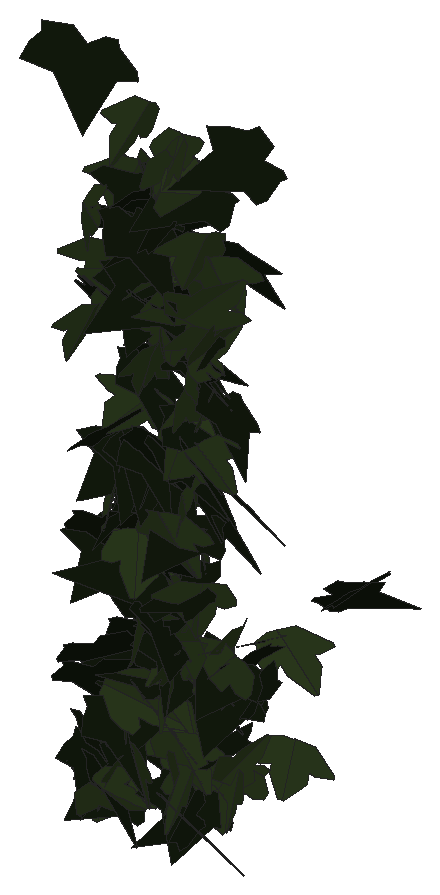
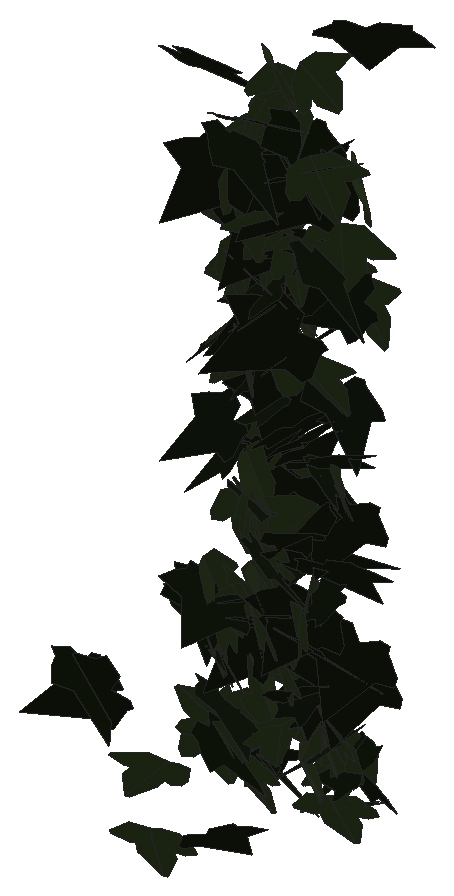
# SketchUp Ruby script. Lengths in inches.
U = 1.inch
M = Sketchup.active_model
def pt(a) = Geom::Point3d.new(a.map { |v| v * U })
def face(e, loops, mat)
  f = e.add_face(loops[0].map { |a| pt(a) })
  loops[1..].each { |l| e.add_face(l.map { |a| pt(a) }).erase! }
  f.material = f.back_material = mat if mat
  f
end
# faces: each face lists its corners as indices into pts; further lists are holes
def faces(e, pts, list, mat = nil) = list.each { |f| face(e, (f[0].is_a?(Array) ? f : [f]).map { |l| l.map { |i| pts[i] } }, mat) }
# xy, xz, yz: faces in a plane at the given z, y or x. An outline is a flat list of corners, or four numbers for a rectangle; further outlines are holes
def ring(l) = l.size == 4 ? [[l[0], l[1]], [l[2], l[1]], [l[2], l[3]], [l[0], l[3]]] : l.each_slice(2).to_a
def flat(e, list, mat, &to3) = list.each { |f| face(e, (f[0].is_a?(Array) ? f : [f]).map { |l| ring(l).map { |u, v| to3.(u, v) } }, mat) }
def xy(e, z, list, mat = nil) = flat(e, list, mat) { |x, y| [x, y, z] }
def xz(e, y, list, mat = nil) = flat(e, list, mat) { |x, z| [x, y, z] }
def yz(e, x, list, mat = nil) = flat(e, list, mat) { |y, z| [x, y, z] }
def lines(e, pts, list) = list.each { |a, b| e.add_line(pt(pts[a]), pt(pts[b])) }
# prism: a flat outline (further loops are holes) pulled along v
def prism(e, loops, v, mat = nil)
  f = face(e, loops, mat); d = Geom::Vector3d.new(v.map { |x| x * U })
  f.pushpull(f.normal.samedirection?(d) ? d.length : -d.length)
end
def box(e, o, s, mat = nil) = prism(e, [[o, [o[0] + s[0], o[1], o[2]], [o[0] + s[0], o[1] + s[1], o[2]], [o[0], o[1] + s[1], o[2]]]], [0, 0, s[2]], mat)
def at(x, y, z, deg = 0) = Geom::Transformation.translation(pt([x, y, z])) * Geom::Transformation.rotation(ORIGIN, Z_AXIS, deg.degrees)
def axes(o, x, y, z) = Geom::Transformation.new([*x, 0, *y, 0, *z, 0, *pt(o).to_a, 1])
def part(name) = M.definitions.add(name)
# library, detail: a bought-in or finely detailed component or shape, given as its bounding box
def library(name, o, s) = part(name).tap { |d| box(d.entities, o, s) }
def detail(e, o, s) = box(e.add_group.entities, o, s)
def put(e, d, t, mat = nil) = e.add_instance(d, t).tap { |i| i.material = mat if mat }
def group(e, t, mat = nil) = e.add_group.tap { |g| g.transformation = t; g.material = mat if mat }.entities
root = M.entities
M.materials.add("1026 AP 7946 SUNNY SIDE UP").color = [254, 231, 186]
M.materials.add("efeu1").color = [18, 25, 13]
M.materials.add("efeu2").color = [43, 57, 29]
c1 = part("ivyleaf_10")
p = [[0,0.5,-0.03],[-0.0625,2.02,-0.43],[-0.19,2.01,-0.46],[-0.54,1.05,-0.29],[-0.52,0.625,-0.18],[-0.83,0.76,-0.28],
  [-1.16,0.64,-0.33],[-1.15,0.33,-0.24],[-0.77,-0.39,0.02],[-0.3,-0.51,0.16],[0.04,-0.48,0.23],[-0.02,2.01,-0.4375],
  [-0.06,2.01,-0.43],[0.04,-0.49,0.23],[0.67,-0.49,0.14],[1.38,0.36,-0.2],[1.375,0.51,-0.24],[0.81,0.65,-0.19],
  [0.62,0.59,-0.15],[0.6,1.09,-0.28],[0.5,1.23,-0.31]]
faces(c1.entities,p,[[0,1,2,3,4,5,6,7,8,9,10],[11,12,0,13,14,15,16,17,18,19,20]],"efeu2")
c2 = part("ivyleaf_9")
p = [[1.54,2.16,1.25],[1.36,2.04,1.19],[-0.21,0.99,0.68],[-0.71,1.11,0.82],[-0.85,0.86,0.67],[-0.8,0.17,0.21],
  [-0.9,-0.01,0.1],[-0.67,-0.16,-0.02],[-0.08,-0.08,-0.05],[-0.03,-0.6,-0.4],[0.65,-0.88,-0.66],[0.83,-0.6,-0.49],
  [1.29,-0.42,-0.43],[1.8125,-0.07,-0.26],[1.21,0.44,0.15]]
faces(c2.entities,p,[[0,1,2,3,4,5,6,7,8,9,10,11,12,13,14]],"efeu1")
put(root,c1,axes([132.02,212.25,286.58],[-0.05135,-0.32161,0.09577],[-0.00011,-0.09523,-0.33345],[0.52721,-0.03135,0.00926]),"1026 AP 7946 SUNNY SIDE UP")
put(root,c2,axes([131.72,212.72,280.17],[0.23766,-0.27259,0.07051],[0.04751,-0.06328,-0.32145],[0.43998,0.15408,-0.00338]),"1026 AP 7946 SUNNY SIDE UP")
put(root,c2,axes([131.95,212.53,280.05],[-0.36569,-0.03792,-0.21571],[0.33427,-0.04152,-0.23598],[-0.00004,-0.31003,0.05612]),"1026 AP 7946 SUNNY SIDE UP")
put(root,c2,axes([131.95,212.3,290.48],[-0.32441,-0.28353,-0.12306],[0.1362,0.08246,-0.36015],[0.46319,-0.22283,0.01971]),"1026 AP 7946 SUNNY SIDE UP")
put(root,c2,axes([132.16,212.8125,282.98],[-0.45442,-0.14963,-0.00161],[0.02273,-0.02637,-0.33398],[0.23418,-0.28779,0.02929]),"1026 AP 7946 SUNNY SIDE UP")
put(root,c1,axes([132.15,212.54,280.18],[-0.41934,0.16198,0.05456],[-0.10293,-0.00838,-0.31876],[-0.24692,-0.27159,0.04022]),"1026 AP 7946 SUNNY SIDE UP")
put(root,c2,axes([132.0625,212.35,281.6875],[0.31074,0.29545,0.0152],[0.03651,0.00018,-0.36565],[-0.46358,0.19805,-0.01861]),"1026 AP 7946 SUNNY SIDE UP")
put(root,c2,axes([132.08,212.34,281.35],[0.36124,0.26486,-0.06174],[-0.0379,-0.06028,-0.36091],[-0.42584,0.23004,-0.02026]),"1026 AP 7946 SUNNY SIDE UP")
put(root,c2,axes([132.36,212.8125,287.3125],[-0.22975,0.30735,-0.01552],[-0.01057,-0.02179,-0.35036],[-0.48389,-0.14546,0.01502]),"1026 AP 7946 SUNNY SIDE UP")
put(root,c1,axes([132.12,212.73,279.58],[0.44585,0.09317,-0.07707],[-0.09975,-0.04747,-0.30671],[-0.15984,0.28952,-0.02357]),"1026 AP 7946 SUNNY SIDE UP")
put(root,c2,axes([132.21,212.71,279.47],[-0.35832,-0.15308,0.14069],[-0.03993,-0.1826,-0.25397],[0.321,-0.19359,0.12545]),"1026 AP 7946 SUNNY SIDE UP")
put(root,c1,axes([132.22,212.48,287.49],[-0.44394,-0.20665,0.02238],[0.00129,-0.03973,-0.35912],[0.32693,-0.28046,0.03181]),"1026 AP 7946 SUNNY SIDE UP")
put(root,c1,axes([131.95,212.37,288.07],[-0.01995,-0.10709,-0.34621],[0.18955,-0.31671,0.09761],[-0.52023,-0.11128,0.04884]),"1026 AP 7946 SUNNY SIDE UP")
put(root,c2,axes([131.85,212.55,286.74],[0.47745,-0.13961,0.0747],[0.09659,-0.04177,-0.34431],[0.22835,0.30956,-0.01056]),"1026 AP 7946 SUNNY SIDE UP")
put(root,c2,axes([131.97,212.81,280.53],[0.25597,-0.24314,-0.1334],[-0.01892,0.14245,-0.29343],[0.43172,0.1504,0.06623]),"1026 AP 7946 SUNNY SIDE UP")
put(root,c2,axes([132.26,215.04,280.1],[-0.30286,-0.23342,0.06508],[-0.05105,-0.05678,-0.3119],[0.37735,-0.19502,0.01004]),"1026 AP 7946 SUNNY SIDE UP")
put(root,c1,axes([132.32,212.83,288.57],[-0.30014,-0.2696,0.11055],[-0.02946,-0.11852,-0.33699],[0.4562,-0.18502,0.05097]),"1026 AP 7946 SUNNY SIDE UP")
put(root,c1,axes([132.21,212.7,280.64],[0.36739,-0.19883,0.07693],[0.06638,-0.06703,-0.31556],[0.32794,0.23632,-0.02231]),"1026 AP 7946 SUNNY SIDE UP")
put(root,c1,axes([132.19,212.5625,284.08],[0.26307,-0.2541,0.13388],[0.12807,-0.1036,-0.31385],[0.43119,0.1858,0.01154]),"1026 AP 7946 SUNNY SIDE UP")
put(root,c2,axes([132.39,212.81,284.39],[-0.37529,-0.19569,0.12924],[-0.06844,-0.14054,-0.30925],[0.36,-0.23072,0.07593]),"1026 AP 7946 SUNNY SIDE UP")
put(root,c2,axes([132.23,212.34,283.59],[0.40729,0.2018,-0.06657],[-0.05299,-0.06335,-0.33734],[-0.3295,0.25963,-0.02804]),"1026 AP 7946 SUNNY SIDE UP")
put(root,c2,axes([132.45,212.13,285.125],[0.01756,0.35128,0.00473],[-0.00169,0.00264,-0.36206],[-0.55237,0.01116,0.00126]),"1026 AP 7946 SUNNY SIDE UP")
put(root,c1,axes([132.54,212.4,287.0625],[-0.46318,-0.07603,0.15402],[-0.20051,-0.09607,-0.30884],[0.17226,-0.31626,0.05466]),"1026 AP 7946 SUNNY SIDE UP")
put(root,c1,axes([132.35,212.98,280.15],[0.22755,-0.24323,0.13062],[0.08195,-0.11795,-0.2919],[0.42447,0.15316,-0.01367]),"1026 AP 7946 SUNNY SIDE UP")
put(root,c1,axes([132.38,212.7,280.51],[-0.06852,0.28961,-0.11758],[-0.02646,-0.11891,-0.30061],[-0.4897,-0.0341,0.03269]),"1026 AP 7946 SUNNY SIDE UP")
put(root,c2,axes([132.17,212.6,282.51],[0.36831,-0.22817,-0.05604],[-0.03262,0.05459,-0.33562],[0.36691,0.23389,0.02641]),"1026 AP 7946 SUNNY SIDE UP")
put(root,c1,axes([132.48,212.3,280.1],[0.14974,-0.29281,0.1003],[0.03245,-0.09736,-0.3176],[0.48494,0.09693,-0.00972]),"1026 AP 7946 SUNNY SIDE UP")
put(root,c2,axes([132.24,212.32,279.87],[0.17493,-0.28596,0.10045],[0.03627,-0.0973,-0.31638],[0.47451,0.11286,-0.01285]),"1026 AP 7946 SUNNY SIDE UP")
put(root,c2,axes([132.36,212.47,280.75],[-0.00677,-0.32176,-0.09337],[-0.00453,0.08884,-0.33096],[0.52483,-0.00338,-0.00406]),"1026 AP 7946 SUNNY SIDE UP")
put(root,c1,axes([132.76,212.55,285.47],[-0.39866,-0.08442,0.21242],[-0.22566,-0.17792,-0.25729],[0.26889,-0.27448,0.09901]),"1026 AP 7946 SUNNY SIDE UP")
put(root,c2,axes([132.93,212.65,281.57],[-0.44466,0.1018,0.12948],[-0.21294,-0.01268,-0.30479],[-0.13778,-0.30897,0.05316]),"1026 AP 7946 SUNNY SIDE UP")
put(root,c1,axes([132.44,211.96,279.91],[-0.20154,-0.17471,-0.26525],[0.26771,0.19242,-0.22155],[0.40798,-0.21257,0.01435]),"1026 AP 7946 SUNNY SIDE UP")
put(root,c1,axes([132.65,212.82,282.05],[-0.36112,0.22578,0.02973],[-0.08714,-0.01754,-0.32767],[-0.34687,-0.23065,0.05137]),"1026 AP 7946 SUNNY SIDE UP")
put(root,c2,axes([132.68,212.48,284.1875],[-0.37109,0.09266,-0.2236],[0.26451,-0.15026,-0.25478],[-0.26135,-0.28365,0.05962]),"1026 AP 7946 SUNNY SIDE UP")
put(root,c2,axes([132.57,212.71,284.49],[-0.16532,-0.3031,0.0933],[-0.0495,-0.08676,-0.33101],[0.49574,-0.10974,-0.00194]),"1026 AP 7946 SUNNY SIDE UP")
put(root,c2,axes([133.03,212.61,282.82],[-0.3856,-0.01037,0.27824],[-0.4146,-0.07134,-0.24982],[0.09384,-0.35781,0.03957]),"1026 AP 7946 SUNNY SIDE UP")
put(root,c2,axes([132.61,212.81,288.4],[-0.29764,-0.27188,0.10545],[0.01456,-0.1295,-0.33248],[0.45742,-0.17279,0.0792]),"1026 AP 7946 SUNNY SIDE UP")
put(root,c1,axes([132.67,212.5,289.67],[-0.0965,-0.28665,0.21499],[0.04521,-0.21673,-0.29693],[0.5572,-0.03206,0.06133]),"1026 AP 7946 SUNNY SIDE UP")
put(root,c2,axes([132.63,212.87,281.05],[-0.2855,-0.26169,0.00417],[0.05023,-0.02884,-0.32534],[0.4085,-0.17935,0.04292]),"1026 AP 7946 SUNNY SIDE UP")
put(root,c2,axes([132.54,212.37,288.24],[0.44916,0.20282,0.03128],[0.06749,-0.01022,-0.35936],[-0.31506,0.28696,-0.03239]),"1026 AP 7946 SUNNY SIDE UP")
put(root,c2,axes([132.59,212.61,282.09],[0.39357,0.21173,0.01409],[0.04462,-0.01431,-0.33648],[-0.33051,0.2502,-0.02865]),"1026 AP 7946 SUNNY SIDE UP")
put(root,c2,axes([132.92,212.3125,288.7],[0.02627,0.34811,-0.02125],[0.00129,-0.02267,-0.35916],[-0.54852,0.01662,-0.00186]),"1026 AP 7946 SUNNY SIDE UP")
put(root,c2,axes([132.68,212.7,284.57],[-0.11155,-0.31917,0.08866],[-0.00763,-0.08886,-0.33704],[0.52048,-0.06971,0.01406]),"1026 AP 7946 SUNNY SIDE UP")
put(root,c1,axes([132.72,212.41,283.38],[0.34118,0.25212,-0.04792],[-0.0265,-0.04866,-0.34242],[-0.40267,0.21682,-0.01807]),"1026 AP 7946 SUNNY SIDE UP")
put(root,c2,axes([132.55,212.67,281.03],[0.40568,-0.18479,-0.0143],[-0.03477,-0.00888,-0.32633],[0.28918,0.25817,-0.01918]),"1026 AP 7946 SUNNY SIDE UP")
put(root,c1,axes([132.8,212.47,288.87],[-0.26253,0.3004,0.00141],[-0.01415,-0.00539,-0.35392],[-0.47213,-0.16688,0.00982]),"1026 AP 7946 SUNNY SIDE UP")
put(root,c1,axes([132.41,212.43,281.05],[0.08597,0.06552,0.35402],[0.51308,0.11482,-0.07544],[-0.19672,0.32809,-0.04206]),"1026 AP 7946 SUNNY SIDE UP")
put(root,c1,axes([132.88,212.57,287.12],[-0.14141,-0.3283,-0.00579],[0.02702,-0.00082,-0.35025],[0.51554,-0.09001,0.01677]),"1026 AP 7946 SUNNY SIDE UP")
put(root,c1,axes([132.65,212.53,282.02],[0.0263,0.01348,0.37394],[0.3193,-0.30153,0.00013],[0.4734,0.20263,-0.02086]),"1026 AP 7946 SUNNY SIDE UP")
put(root,c2,axes([132.84,212.61,287.16],[-0.28808,-0.28899,0.02913],[0.00038,-0.03552,-0.35216],[0.45684,-0.18221,0.01866]),"1026 AP 7946 SUNNY SIDE UP")
put(root,c1,axes([132.63,212.6,283.5],[0.33728,0.20601,0.16568],[0.18093,0.11068,-0.30574],[-0.36772,0.24342,0.00154]),"1026 AP 7946 SUNNY SIDE UP")
put(root,c2,axes([133.09,212.47,287.2],[-0.48227,-0.13072,0.09985],[-0.11533,-0.07531,-0.34157],[0.2292,-0.31295,0.03823]),"1026 AP 7946 SUNNY SIDE UP")
put(root,c2,axes([132.6875,212.68,285.83],[0.04918,-0.34284,0.00206],[-0.00195,-0.00407,-0.35467],[0.53911,0.03126,-0.00147]),"1026 AP 7946 SUNNY SIDE UP")
put(root,c2,axes([132.66,212.6,288.14],[0.50373,0.14468,0.03593],[0.07065,-0.01713,-0.36053],[-0.22277,0.32171,-0.03309]),"1026 AP 7946 SUNNY SIDE UP")
put(root,c1,axes([132.83,212.24,280.37],[-0.27438,0.24669,-0.08135],[0.04041,-0.07994,-0.31075],[-0.40596,-0.1747,0.02405]),"1026 AP 7946 SUNNY SIDE UP")
put(root,c2,axes([132.55,212.67,283.3],[0.12724,-0.13399,0.34566],[0.25159,-0.29587,-0.16284],[0.5106,0.17917,-0.0059]),"1026 AP 7946 SUNNY SIDE UP")
put(root,c2,axes([132.77,212.72,284.71],[-0.01177,-0.3344,-0.05727],[-0.00083,0.05372,-0.34426],[0.53254,-0.00731,-0.0018]),"1026 AP 7946 SUNNY SIDE UP")
put(root,c1,axes([132.88,212.86,281.38],[0.33985,-0.23052,0.05338],[0.06294,-0.03528,-0.32571],[0.36661,0.21975,0.00644]),"1026 AP 7946 SUNNY SIDE UP")
put(root,c1,axes([132.87,212.89,280.42],[0.18134,0.28609,-0.04332],[-0.01355,-0.0436,-0.31792],[-0.45486,0.11536,-0.0078]),"1026 AP 7946 SUNNY SIDE UP")
put(root,c2,axes([132.7,212.82,286.125],[0.49959,0.14204,0.13463],[0.20268,0.02912,-0.35749],[-0.22474,0.34201,-0.02312]),"1026 AP 7946 SUNNY SIDE UP")
put(root,c2,axes([132.66,212.57,283.43],[-0.0276,0.01244,0.34803],[0.36805,-0.24354,0.02034],[0.38338,0.23469,0.00552]),"1026 AP 7946 SUNNY SIDE UP")
put(root,c1,axes([133.07,212.23,286.4],[-0.00791,-0.34904,-0.0091],[0.00657,0.00679,-0.35955],[0.5489,-0.00511,0.00417]),"1026 AP 7946 SUNNY SIDE UP")
put(root,c2,axes([132.83,212.19,288.26],[0.11329,-0.34626,-0.11686],[-0.00785,0.11268,-0.36326],[0.57192,0.07014,0.01816]),"1026 AP 7946 SUNNY SIDE UP")
put(root,c2,axes([132.67,212.43,286.79],[0.48405,-0.08066,0.14025],[0.18948,-0.07502,-0.32586],[0.16221,0.32832,-0.03787]),"1026 AP 7946 SUNNY SIDE UP")
put(root,c2,axes([133.28,212.27,288.38],[-0.39014,0.19727,-0.1389],[0.11506,-0.12396,-0.32362],[-0.35871,-0.25431,0.04726]),"1026 AP 7946 SUNNY SIDE UP")
put(root,c1,axes([133.04,212.96,280.76],[0.06671,-0.3104,-0.01636],[0.00849,-0.01351,0.32265],[-0.48851,-0.04262,0.00337]),"1026 AP 7946 SUNNY SIDE UP")
put(root,c1,axes([133,212.86,287.63],[0.28652,0.28795,0.03353],[0.04248,0.01946,-0.3507],[-0.45339,0.1838,-0.01167]),"1026 AP 7946 SUNNY SIDE UP")
put(root,c2,axes([133.15,212.37,285.04],[0.45515,0.12855,-0.14607],[-0.1758,-0.09668,-0.32434],[-0.2453,0.30782,-0.03858]),"1026 AP 7946 SUNNY SIDE UP")
put(root,c2,axes([133.45,212.61,282.7],[-0.36608,0.23419,-0.01894],[-0.00426,-0.03042,-0.33952],[-0.36952,-0.23166,0.02268]),"1026 AP 7946 SUNNY SIDE UP")
put(root,c1,axes([133,215.08,280.83],[0.31959,0.20062,0.14624],[0.1968,0.07233,-0.29185],[-0.33136,0.23644,-0.03229]),"1026 AP 7946 SUNNY SIDE UP")
put(root,c1,axes([133.23,212.19,286.54],[0.09641,-0.29838,-0.17621],[0.06062,0.17694,-0.30574],[0.53606,0.03365,0.06626]),"1026 AP 7946 SUNNY SIDE UP")
put(root,c1,axes([133.23,212.85,281.76],[0.32329,-0.24763,-0.01854],[0.0259,0.03511,-0.3294],[0.38938,0.20326,0.0373]),"1026 AP 7946 SUNNY SIDE UP")
put(root,c1,axes([133.3125,212.86,284.08],[-0.00162,-0.32701,0.04336],[-0.00702,-0.04393,-0.33711],[0.51876,-0.00162,-0.00443]),"1026 AP 7946 SUNNY SIDE UP")
put(root,c1,axes([133.5,212.43,282.22],[0.28332,-0.06038,-0.27638],[-0.32867,0.17774,-0.18503],[0.28016,0.26956,0.06244]),"1026 AP 7946 SUNNY SIDE UP")
put(root,c2,axes([133.02,212.77,286.4],[0.22117,-0.29926,-0.09639],[0.00006,0.10073,-0.33739],[0.49223,0.13445,0.04335]),"1026 AP 7946 SUNNY SIDE UP")
put(root,c1,axes([133.27,212.56,287.23],[-0.15771,-0.33258,-0.04397],[0.09241,0.02446,-0.35416],[0.5187,-0.10548,0.04972]),"1026 AP 7946 SUNNY SIDE UP")
put(root,c2,axes([133.27,212.83,281.83],[-0.32737,-0.24699,-0.00352],[0.06004,-0.02958,-0.32922],[0.38371,-0.20609,0.04851]),"1026 AP 7946 SUNNY SIDE UP")
put(root,c1,axes([133.36,212.36,281.97],[0.02794,-0.32837,-0.10644],[-0.02402,0.10074,-0.33805],[0.53988,0.02147,-0.00953]),"1026 AP 7946 SUNNY SIDE UP")
put(root,c2,axes([133.125,212.52,282.26],[-0.06001,-0.26996,0.20533],[0.06915,-0.2044,-0.27562],[0.52454,-0.00394,0.05982]),"1026 AP 7946 SUNNY SIDE UP")
put(root,c2,axes([133,212.74,286.67],[0.30951,-0.28317,0.01911],[0.04012,-0.00678,-0.35488],[0.44458,0.19775,0.01872]),"1026 AP 7946 SUNNY SIDE UP")
put(root,c1,axes([133.17,212.44,281.53],[0.28084,-0.1946,0.18575],[0.19,-0.13532,-0.27289],[0.37268,0.21563,-0.00085]),"1026 AP 7946 SUNNY SIDE UP")
put(root,c1,axes([133.4,212.33,286.92],[-0.42699,-0.20649,0.02993],[-0.01226,-0.03954,-0.3506],[0.32791,-0.27035,0.02587]),"1026 AP 7946 SUNNY SIDE UP")
put(root,c2,axes([133.0625,212.68,286.16],[0.52825,-0.08164,0.00723],[0.00112,-0.02865,-0.35519],[0.1289,0.33481,-0.02654]),"1026 AP 7946 SUNNY SIDE UP")
put(root,c2,axes([133.59,212.9,288.625],[-0.17487,0.32529,-0.03444],[-0.01255,-0.03994,-0.35377],[-0.51434,-0.10962,0.02034]),"1026 AP 7946 SUNNY SIDE UP")
put(root,c1,axes([133.26,212.64,280.52],[-0.44557,-0.06004,-0.11776],[0.19649,-0.06127,-0.28719],[0.04917,-0.29922,0.08054]),"1026 AP 7946 SUNNY SIDE UP")
put(root,c1,axes([133.29,212.37,289.3125],[-0.1644,-0.29117,-0.2125],[0.19161,0.17108,-0.31395],[0.52576,-0.1534,0.04796]),"1026 AP 7946 SUNNY SIDE UP")
put(root,c2,axes([133.1,212.5,284.92],[0.32812,-0.25188,-0.09606],[-0.02957,0.10231,-0.33258],[0.42051,0.20373,0.05157]),"1026 AP 7946 SUNNY SIDE UP")
put(root,c1,axes([133.36,212.36,289.45],[0.37341,-0.26371,0.03526],[0.00857,-0.04304,-0.36496],[0.41836,0.23626,-0.02399]),"1026 AP 7946 SUNNY SIDE UP")
put(root,c2,axes([133.28,212.47,287.23],[0.32044,0.25277,0.11024],[0.11616,0.076,-0.33391],[-0.41477,0.21657,-0.00834]),"1026 AP 7946 SUNNY SIDE UP")
put(root,c1,axes([133.4,212.7,282.21],[0.23272,-0.29533,0.01306],[-0.00202,-0.0167,-0.3403],[0.46493,0.14776,-0.00801]),"1026 AP 7946 SUNNY SIDE UP")
put(root,c2,axes([133.69,212.67,286.72],[-0.4756,0.17076,-0.00236],[-0.01941,-0.02846,-0.35658],[-0.26785,-0.30114,0.03002]),"1026 AP 7946 SUNNY SIDE UP")
put(root,c1,axes([133.47,212.19,280.3],[0.16899,-0.25811,-0.19591],[-0.06551,0.18608,-0.28556],[0.49847,0.11196,0.02889]),"1026 AP 7946 SUNNY SIDE UP")
put(root,c2,axes([133.64,212.39,279.7],[-0.40245,0.17614,-0.03907],[0.03322,-0.03783,-0.3197],[-0.28169,-0.25611,0.01812]),"1026 AP 7946 SUNNY SIDE UP")
put(root,c1,axes([133.5,212.83,279.74],[0.42305,-0.12728,-0.10434],[-0.1553,0.02595,-0.30592],[0.20233,0.28605,-0.01666]),"1026 AP 7946 SUNNY SIDE UP")
put(root,c2,axes([133.61,212.7,288.79],[-0.51234,-0.1106,0.06176],[-0.01869,-0.14016,-0.33029],[0.1974,-0.30032,0.12903]),"1026 AP 7946 SUNNY SIDE UP")
put(root,c1,axes([133.48,212.4375,282.82],[0.37271,-0.20599,-0.11165],[-0.06278,0.11476,-0.31743],[0.3597,0.23347,0.06028]),"1026 AP 7946 SUNNY SIDE UP")
put(root,c2,axes([133.44,212.67,279.81],[-0.29395,-0.25273,-0.01862],[0.03919,0.00222,-0.32326],[0.39631,-0.18767,0.01816]),"1026 AP 7946 SUNNY SIDE UP")
put(root,c1,axes([133.4,214.71,279.54],[0.47351,0.07925,-0.01677],[-0.01939,-0.01879,-0.32053],[-0.12587,0.30102,-0.0137]),"1026 AP 7946 SUNNY SIDE UP")
put(root,c1,axes([133.3,212.55,281.5],[0.47852,0.05678,0.0851],[0.11727,0.04665,-0.31704],[-0.10469,0.31178,0.03387]),"1026 AP 7946 SUNNY SIDE UP")
put(root,c2,axes([133.29,212.84,281.5],[0.47461,-0.0762,-0.07099],[-0.11359,-0.00725,-0.31978],[0.11422,0.30942,-0.02306]),"1026 AP 7946 SUNNY SIDE UP")
put(root,c1,axes([133.41,212.16,284.02],[-0.4909,0.02305,-0.12555],[0.18611,-0.04446,-0.32094],[-0.05896,-0.33223,0.03225]),"1026 AP 7946 SUNNY SIDE UP")
put(root,c2,axes([133.62,212.42,284.08],[-0.5107,-0.11036,-0.06163],[0.10747,-0.01832,-0.35123],[0.16502,-0.32963,0.038]),"1026 AP 7946 SUNNY SIDE UP")
put(root,c1,axes([133.57,212.6875,283.51],[-0.19314,0.30329,0.06685],[-0.12564,0.03464,-0.33119],[-0.47065,-0.13371,0.06098]),"1026 AP 7946 SUNNY SIDE UP")
put(root,c1,axes([133.35,212.33,288.84],[-0.03546,-0.12883,-0.35893],[0.31545,0.28868,-0.12191],[0.49029,-0.19506,0.05248]),"1026 AP 7946 SUNNY SIDE UP")
put(root,c1,axes([133.65,212.72,281.95],[-0.2328,-0.27053,0.08724],[-0.03976,-0.08429,-0.31768],[0.4447,-0.14916,0.01727]),"1026 AP 7946 SUNNY SIDE UP")
put(root,c2,axes([133.77,212.8,280.47],[-0.00762,0.27094,0.16054],[-0.13198,0.14749,-0.26865],[-0.47216,-0.0456,0.0725]),"1026 AP 7946 SUNNY SIDE UP")
put(root,c1,axes([133.59,212.74,285.6875],[0.1981,-0.31343,-0.05496],[-0.00333,0.05465,-0.34717],[0.49945,0.12468,0.01949]),"1026 AP 7946 SUNNY SIDE UP")
put(root,c1,axes([133.5625,212.39,285.4],[0.18187,0.27477,-0.18631],[-0.11607,-0.16683,-0.30809],[-0.50543,0.13718,0.00371]),"1026 AP 7946 SUNNY SIDE UP")
put(root,c2,axes([133.78,213.07,280.2],[-0.23938,0.21814,-0.16677],[0.09606,-0.15477,-0.27286],[-0.4174,-0.16073,0.03285]),"1026 AP 7946 SUNNY SIDE UP")
put(root,c2,axes([133.91,212.29,283.19],[-0.39891,0.20464,-0.01167],[-0.028,-0.04178,-0.333],[-0.32115,-0.25054,0.04352]),"1026 AP 7946 SUNNY SIDE UP")
put(root,c1,axes([133.68,212.85,281.73],[-0.02244,-0.30518,0.09637],[0.02297,-0.09589,-0.31474],[0.50218,-0.00925,0.0187]),"1026 AP 7946 SUNNY SIDE UP")
put(root,c1,axes([133.61,212.22,280.27],[0.34092,-0.25567,0.10086],[0.07214,-0.09106,-0.34507],[0.42522,0.22042,-0.02232]),"1026 AP 7946 SUNNY SIDE UP")
put(root,c1,axes([133.82,213.03,280.09],[-0.40844,-0.13873,0.10179],[-0.08541,-0.10475,-0.2969],[0.25459,-0.25772,0.06369]),"1026 AP 7946 SUNNY SIDE UP")
put(root,c1,axes([133.75,212.52,286.82],[-0.18667,-0.32068,-0.02533],[0.02551,0.01826,-0.35205],[0.50487,-0.1195,0.00842]),"1026 AP 7946 SUNNY SIDE UP")
put(root,c1,axes([133.76,212.61,287.82],[-0.06217,-0.34101,0.03391],[-0.00148,-0.03497,-0.35385],[0.539,-0.03943,0.00294]),"1026 AP 7946 SUNNY SIDE UP")
put(root,c2,axes([133.375,212.4,279.68],[0.31876,-0.21033,0.11175],[0.1473,-0.06154,-0.30035],[0.34267,0.22211,0.02516]),"1026 AP 7946 SUNNY SIDE UP")
put(root,c1,axes([133.58,212.98,281.18],[0.25398,-0.15769,0.22515],[0.21405,-0.17337,-0.23258],[0.36706,0.21021,-0.02016]),"1026 AP 7946 SUNNY SIDE UP")
put(root,c2,axes([133.54,212.48,285.44],[0.09341,-0.33237,-0.05681],[-0.01656,0.05222,-0.34752],[0.52903,0.06032,-0.00085]),"1026 AP 7946 SUNNY SIDE UP")
put(root,c1,axes([133.6,212.3,284.41],[-0.0652,-0.12015,-0.32167],[0.12221,-0.30881,0.11022],[-0.51065,-0.05856,0.06745]),"1026 AP 7946 SUNNY SIDE UP")
put(root,c1,axes([133.84,212.29,283.11],[-0.3664,-0.22765,0.00823],[0.0189,-0.02554,-0.33463],[0.35776,-0.2318,0.02611]),"1026 AP 7946 SUNNY SIDE UP")
put(root,c1,axes([133.87,212.26,288.28],[-0.20352,-0.3213,0.0736],[-0.01218,-0.07573,-0.35666],[0.51804,-0.12801,0.02053]),"1026 AP 7946 SUNNY SIDE UP")
put(root,c1,axes([133.76,212.1,286.09],[0.06465,-0.27573,-0.21589],[0.10324,0.21188,-0.27476],[0.53318,-0.0076,0.07938]),"1026 AP 7946 SUNNY SIDE UP")
put(root,c1,axes([133.82,212.34,286.5],[0.06346,-0.11467,0.35808],[-0.08916,0.34417,0.12554],[-0.56955,-0.06665,0.02025]),"1026 AP 7946 SUNNY SIDE UP")
put(root,c1,axes([133.83,212.98,281.4],[0.1949,-0.28176,0.07036],[0.03038,-0.06783,-0.31736],[0.45546,0.1251,-0.00894]),"1026 AP 7946 SUNNY SIDE UP")
put(root,c2,axes([133.64,212.73,284.17],[0.35685,-0.21206,-0.12146],[-0.12777,0.08394,-0.31944],[0.35851,0.24099,0.00705]),"1026 AP 7946 SUNNY SIDE UP")
put(root,c2,axes([133.85,212.89,282.03],[0.27559,0.2419,0.12125],[-0.01396,0.14407,-0.29403],[-0.42182,0.15327,0.08895]),"1026 AP 7946 SUNNY SIDE UP")
put(root,c1,axes([134.1,212.56,282.04],[-0.42258,0.08139,0.16439],[-0.27989,-0.09623,-0.25959],[-0.02511,-0.29712,0.12706]),"1026 AP 7946 SUNNY SIDE UP")
put(root,c2,axes([133.89,212.74,281.53],[-0.36473,-0.20138,-0.07587],[0.13854,0.0076,-0.31208],[0.30672,-0.24291,0.05074]),"1026 AP 7946 SUNNY SIDE UP")
put(root,c2,axes([133.92,212.85,281.83],[-0.30189,-0.24218,0.092],[0.01254,-0.11843,-0.30914],[0.40643,-0.17624,0.07787]),"1026 AP 7946 SUNNY SIDE UP")
put(root,c2,axes([134.1,215.22,281.96],[-0.04114,0.31574,-0.02149],[-0.01668,-0.02359,-0.32627],[-0.49747,-0.02532,0.01272]),"1026 AP 7946 SUNNY SIDE UP")
put(root,c1,axes([133.98,212.85,282.3],[0.05025,-0.32107,0.03036],[-0.00013,-0.03145,-0.33257],[0.50724,0.0318,-0.00309]),"1026 AP 7946 SUNNY SIDE UP")
put(root,c2,axes([133.68,212.4,285.06],[0.21944,-0.27787,0.13434],[0.06574,-0.12645,-0.32054],[0.47921,0.14459,-0.01755]),"1026 AP 7946 SUNNY SIDE UP")
put(root,c2,axes([133.72,215.24,281.73],[0.355,0.12087,0.19607],[0.25346,0.10039,-0.26303],[-0.24656,0.27723,0.01191]),"1026 AP 7946 SUNNY SIDE UP")
put(root,c2,axes([133.73,212.8,284.5],[0.48308,-0.12118,-0.03544],[-0.0412,0.02537,-0.33978],[0.19344,0.30803,0.01614]),"1026 AP 7946 SUNNY SIDE UP")
put(root,c1,axes([133.91,212.88,280.2],[-0.09246,-0.25775,0.17459],[0.04351,0.16892,0.27319],[-0.48436,0.06438,-0.00878]),"1026 AP 7946 SUNNY SIDE UP")
put(root,c1,axes([133.82,212.25,287.22],[-0.30733,-0.25878,0.17961],[0.20087,0.12322,0.33386],[-0.44905,0.23222,0.02643]),"1026 AP 7946 SUNNY SIDE UP")
put(root,c1,axes([133.96,212.44,287.88],[-0.47938,-0.12438,-0.10224],[0.15561,0.0178,-0.33848],[0.19504,-0.31991,0.01876]),"1026 AP 7946 SUNNY SIDE UP")
put(root,c1,axes([133.92,212.86,280.1],[0.3375,-0.20485,0.10835],[0.12223,-0.07256,-0.30609],[0.34172,0.22828,0.00248]),"1026 AP 7946 SUNNY SIDE UP")
put(root,c2,axes([134.125,212.77,281.98],[0.07267,0.31873,0.01723],[0.02105,0.01312,-0.3315],[-0.50127,0.04676,-0.01142]),"1026 AP 7946 SUNNY SIDE UP")
put(root,c2,axes([133.84,212.8125,285.7],[0.07573,-0.33098,0.05249],[0.00302,-0.0531,-0.34482],[0.52701,0.04786,-0.00557]),"1026 AP 7946 SUNNY SIDE UP")
put(root,c2,axes([133.87,212.67,288],[0.5436,0.04911,-0.01575],[-0.01912,-0.02486,-0.3591],[-0.07872,0.34517,-0.02155]),"1026 AP 7946 SUNNY SIDE UP")
put(root,c2,axes([134.43,212.77,289.45],[-0.53572,0.01265,0.07614],[-0.11775,-0.0669,-0.34456],[0.00321,-0.34213,0.06811]),"1026 AP 7946 SUNNY SIDE UP")
put(root,c2,axes([134.39,212.75,281.51],[-0.118,0.25096,0.1847],[-0.13404,0.15894,-0.26715],[-0.46472,-0.10957,0.03015]),"1026 AP 7946 SUNNY SIDE UP")
put(root,c1,axes([134.03,212.11,285.3],[-0.24595,-0.25877,-0.16018],[0.21918,0.09163,-0.30389],[0.41973,-0.19948,0.06483]),"1026 AP 7946 SUNNY SIDE UP")
